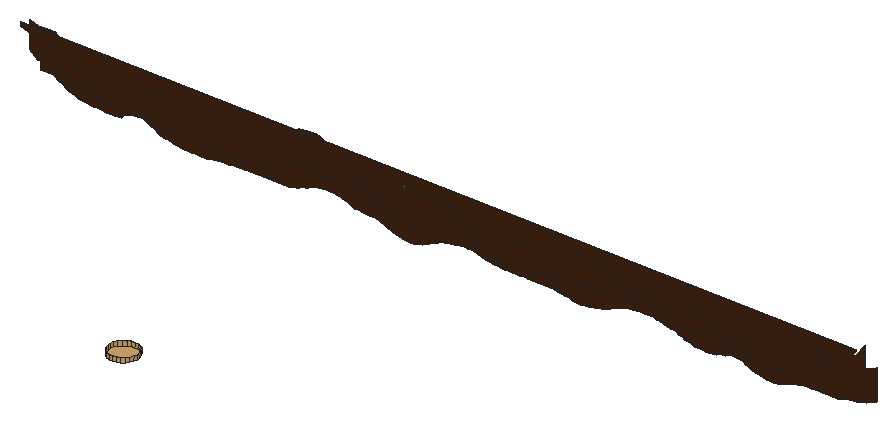
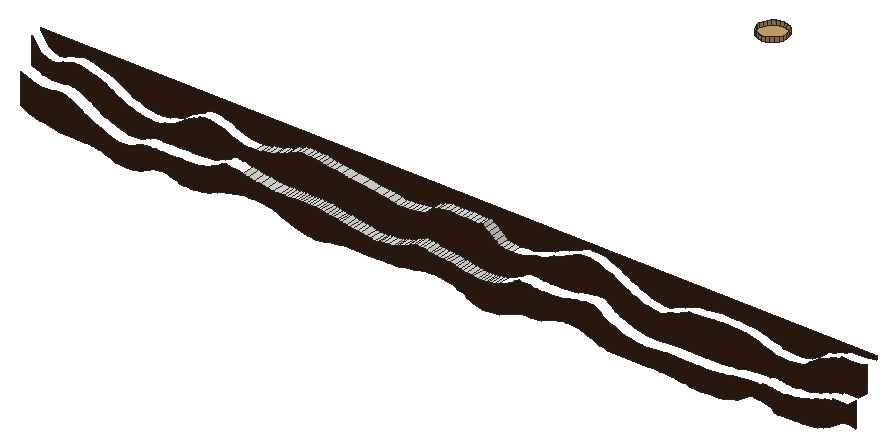
# SketchUp Ruby script. Lengths in inches.
U = 1.inch
M = Sketchup.active_model
def pt(a) = Geom::Point3d.new(a.map { |v| v * U })
def face(e, loops, mat)
  f = e.add_face(loops[0].map { |a| pt(a) })
  loops[1..].each { |l| e.add_face(l.map { |a| pt(a) }).erase! }
  f.material = f.back_material = mat if mat
  f
end
# faces: each face lists its corners as indices into pts; further lists are holes
def faces(e, pts, list, mat = nil) = list.each { |f| face(e, (f[0].is_a?(Array) ? f : [f]).map { |l| l.map { |i| pts[i] } }, mat) }
# xy, xz, yz: faces in a plane at the given z, y or x. An outline is a flat list of corners, or four numbers for a rectangle; further outlines are holes
def ring(l) = l.size == 4 ? [[l[0], l[1]], [l[2], l[1]], [l[2], l[3]], [l[0], l[3]]] : l.each_slice(2).to_a
def flat(e, list, mat, &to3) = list.each { |f| face(e, (f[0].is_a?(Array) ? f : [f]).map { |l| ring(l).map { |u, v| to3.(u, v) } }, mat) }
def xy(e, z, list, mat = nil) = flat(e, list, mat) { |x, y| [x, y, z] }
def xz(e, y, list, mat = nil) = flat(e, list, mat) { |x, z| [x, y, z] }
def yz(e, x, list, mat = nil) = flat(e, list, mat) { |y, z| [x, y, z] }
def lines(e, pts, list) = list.each { |a, b| e.add_line(pt(pts[a]), pt(pts[b])) }
# prism: a flat outline (further loops are holes) pulled along v
def prism(e, loops, v, mat = nil)
  f = face(e, loops, mat); d = Geom::Vector3d.new(v.map { |x| x * U })
  f.pushpull(f.normal.samedirection?(d) ? d.length : -d.length)
end
def box(e, o, s, mat = nil) = prism(e, [[o, [o[0] + s[0], o[1], o[2]], [o[0] + s[0], o[1] + s[1], o[2]], [o[0], o[1] + s[1], o[2]]]], [0, 0, s[2]], mat)
def at(x, y, z, deg = 0) = Geom::Transformation.translation(pt([x, y, z])) * Geom::Transformation.rotation(ORIGIN, Z_AXIS, deg.degrees)
def axes(o, x, y, z) = Geom::Transformation.new([*x, 0, *y, 0, *z, 0, *pt(o).to_a, 1])
def part(name) = M.definitions.add(name)
# library, detail: a bought-in or finely detailed component or shape, given as its bounding box
def library(name, o, s) = part(name).tap { |d| box(d.entities, o, s) }
def detail(e, o, s) = box(e.add_group.entities, o, s)
def put(e, d, t, mat = nil) = e.add_instance(d, t).tap { |i| i.material = mat if mat }
def group(e, t, mat = nil) = e.add_group.tap { |g| g.transformation = t; g.material = mat if mat }.entities
root = M.entities
M.materials.add("[Field Square Tile]").color = [211, 167, 108]
M.materials.add("[Wood Veneer 01]").color = [66, 38, 20]
xy(root,243.05,[[1237.04,2398.8,1237.72,2401.37]])
xy(root,243.07,[[1235.1875,2398.8,1235.77,2401.37]])
xy(root,243.09,[[1231.875,2398.8,1232.4,2401.37],[1232.4,2398.8,1232.92,2401.37],[1232.92,2398.8,1233.58,2401.37],[1233.58,2398.8,1234.03,2401.37]])
xy(root,249.21,[[1204.67,2396.68,1205.56,2398.8]])
xy(root,249.22,[[1206.28,2396.68,1207.1875,2398.8]])
xy(root,249.23,[[1207.83,2396.68,1208.73,2398.8]])
xy(root,250.6875,[[1203.22,2328.39,1202.56,2328.48,1201.94,2328.74,1201.41,2329.14,1201,2329.68,1200.75,2330.29,1200.66,2330.96,1200.75,2331.62,1201,2332.24,1201.41,2332.77,1201.94,2333.18,1202.56,2333.43,1203.22,2333.52,1203.88,2333.43,1204.5,2333.18,1205.03,2332.77,1205.44,2332.24,1205.7,2331.62,1205.78,2330.96,1205.7,2330.29,1205.44,2329.68,1205.03,2329.14,1204.5,2328.74,1203.88,2328.48]],"[Field Square Tile]")
xz(root,2396.68,[[1263.09,244.87,1264,245.01,1264.9375,245.12,1265.7,245.25,1266.46,245.41,1267.09,245.78,1267.89,245.88,1268.6,246.16,1269.2,246.57,1269.99,246.9,1270.59,247.35,1271.26,247.62,1271.85,248.06,1272.61,248.32,1273.72,248.66,1274.5,248.79,1275.36,249.19,1276.03,249.32,1276.96,249.41,1277.81,249.48,1278.56,249.21,1279.2,248.96,1279.9,248.9,1280.7,248.42,1281.41,248.3,1282.12,248.22,1282.9375,248.56,1283.87,249.02,1285.6,251.16,1285.6,251.5,1131.59,251.5,1131.59,250.88,1133.18,250.53,1134.8,250.54,1136.26,250.55,1136.79,250.15,1137.4,249.97,1138.2,249.8,1138.87,249.41,1139.54,249.2,1140.31,249.01,1140.8,248.51,1141.43,248.07,1142.08,247.72,1142.72,247.25,1143.27,246.88,1143.99,246.73,1144.65,246.62,1145.39,246.54,1146.17,246.51,1146.95,246.58,1147.75,246.59,1148.55,246.69,1149.26,247.03,1149.95,247.2,1150.92,247.39,1151.55,247.78,1152.33,247.89,1153.33,248.18,1153.97,248.29,1154.86,248.35,1155.59,248.4,1156.58,248.4375,1157.24,248.46,1158.13,248.47,1158.87,248.48,1159.76,248.49,1160.49,248.39,1161.89,248.28,1162.92,248.15,1163.74,248.11,1164.54,248.08,1165.38,247.66,1166.01,247.46,1166.69,247.08,1167.375,246.94,1168.23,246.66,1168.84,246.35,1169.61,246.05,1170.51,246.13,1171.22,246.29,1172.02,246.41,1172.93,246.55,1173.66,246.92,1174.27,247.12,1174.95,247.31,1175.52,247.71,1176.45,248.03,1177.16,248.46,1177.94,248.82,1178.66,249.37,1179.45,249.5625,1180.35,249.9,1181.27,250.35,1181.93,250.49,1182.74,250.6,1183.76,250.58,1184.4,250.61,1185.02,250.32,1185.71,250.0625,1186.37,249.68,1187.13,249.46,1188.02,248.95,1189.24,248.69,1190.15,248.26,1190.75,247.9,1191.88,247.66,1192.46,247.53,1193.14,247.25,1193.95,246.95,1194.64,246.75,1195.43,246.66,1196.14,246.59,1197.03,246.55,1197.96,246.63,1198.7,246.74,1199.43,246.87,1200.04,247.42,1200.71,247.96,1201.28,248.44,1202.02,248.85,1202.49,249.34,1203.22,249.125,1203.99,249.17,1204.67,249.21,1205.56,249.21,1206.28,249.22,1207.1875,249.22,1207.83,249.23,1208.73,249.23,1209.47,249.24,1210.27,249.14,1210.9,248.82,1211.69,248.54,1212.39,248.04,1213.08,247.48,1213.97,247.29,1214.79,247.15,1215.52,247.05,1216.24,247,1217.15,246.96,1217.875,246.94,1218.79,247.04,1219.85,247.36,1221.03,247.43,1222.68,247.6,1224.66,247.98,1226.86,248.1875,1228.47,248.49,1229.72,248.62,1230.66,248.69,1231.34,248.75,1232,249.09,1232.7,249.18,1233.48,249.13,1234.18,249.17,1234.88,249.18,1235.78,249.29,1236.51,249.21,1237.12,248.8,1237.8125,248.73,1238.59,248.26,1239.29,248.02,1240.09,247.8125,1240.8,247.4,1241.71,247.27,1242.45,247.18,1243.375,246.91,1244.24,246.84,1245.19,246.79,1245.97,246.75,1246.72,246.83,1247.76,247.25,1248.63,247.55,1249.3,247.66,1249.93,248.16,1250.72,248.41,1251.42,248.52,1252.12,248.72,1252.82,248.8,1253.71,248.85,1254.54,248.6875,1255.08,248.26,1255.77,248.06,1256.66,247.55,1257.37,247.19,1258.18,246.63,1258.8125,246.13,1259.4,245.83,1260.08,245.67,1260.95,245.46,1261.66,245.0625,1262.375,244.95]],"[Wood Veneer 01]")
xz(root,2398.8,[[1267.09,241.09,1267.66,241.14,1268.3,241.35,1268.89,241.46,1269.83,241.85,1270.83,242.23,1271.39,242.42,1272.11,242.61,1272.625,242.91,1273,243.14,1273.54,243.52,1274.02,243.71,1274.35,244.02,1274.79,244.21,1275.38,244.57,1275.85,244.76,1276.47,245.125,1276.97,245.32,1277.45,245.41,1278,245.48,1278.49,245.59,1279.02,245.55,1279.63,245.35,1280.12,245.31,1280.67,245.27,1281.23,245.24,1281.79,245.22,1282.35,245.34,1282.98,245.42,1283.5625,245.52,1283.94,245.76,1284.41,245.9,1285.6,246.43,1285.6,251.16,1283.87,249.02,1282.9375,248.56,1282.12,248.22,1281.41,248.3,1280.7,248.42,1279.9,248.9,1279.2,248.96,1278.56,249.21,1277.81,249.48,1276.96,249.41,1276.03,249.32,1275.36,249.19,1274.5,248.79,1273.72,248.66,1272.61,248.32,1271.85,248.06,1271.26,247.62,1270.59,247.35,1269.99,246.9,1269.2,246.57,1268.6,246.16,1267.89,245.88,1267.09,245.78,1266.46,245.41,1265.7,245.25,1264.9375,245.12,1264,245.01,1263.09,244.87,1262.375,244.95,1261.66,245.0625,1260.95,245.46,1260.08,245.67,1259.4,245.83,1258.8125,246.13,1258.18,246.63,1257.37,247.19,1256.66,247.55,1255.77,248.06,1255.08,248.26,1254.54,248.6875,1253.71,248.85,1252.82,248.8,1252.12,248.72,1251.42,248.52,1250.72,248.41,1249.93,248.16,1249.3,247.66,1248.63,247.55,1247.76,247.25,1246.72,246.83,1245.97,246.75,1245.19,246.79,1244.24,246.84,1243.375,246.91,1242.45,247.18,1241.71,247.27,1240.8,247.4,1240.09,247.8125,1239.29,248.02,1238.59,248.26,1237.8125,248.73,1237.12,248.8,1236.51,249.21,1235.78,249.29,1234.88,249.18,1234.18,249.17,1233.48,249.13,1232.7,249.18,1232,249.09,1231.34,248.75,1230.66,248.69,1229.72,248.62,1228.47,248.49,1226.86,248.1875,1224.66,247.98,1222.68,247.6,1221.03,247.43,1219.85,247.36,1218.79,247.04,1217.875,246.94,1217.15,246.96,1216.24,247,1215.52,247.05,1214.79,247.15,1213.97,247.29,1213.08,247.48,1212.39,248.04,1211.69,248.54,1210.9,248.82,1210.27,249.14,1209.47,249.24,1208.73,249.23,1207.83,249.23,1207.1875,249.22,1206.28,249.22,1205.56,249.21,1204.67,249.21,1203.99,249.17,1203.22,249.125,1202.49,249.34,1202.02,248.85,1201.28,248.44,1200.71,247.96,1200.04,247.42,1199.43,246.87,1198.7,246.74,1197.96,246.63,1197.03,246.55,1196.14,246.59,1195.43,246.66,1194.64,246.75,1193.95,246.95,1193.14,247.25,1192.46,247.53,1191.88,247.66,1190.75,247.9,1190.15,248.26,1189.24,248.69,1188.02,248.95,1187.13,249.46,1186.37,249.68,1185.71,250.0625,1185.02,250.32,1184.4,250.61,1183.76,250.58,1182.74,250.6,1181.93,250.49,1181.27,250.35,1180.35,249.9,1179.45,249.5625,1178.66,249.37,1177.94,248.82,1177.16,248.46,1176.45,248.03,1175.52,247.71,1174.95,247.31,1174.27,247.12,1173.66,246.92,1172.93,246.55,1172.02,246.41,1171.22,246.29,1170.51,246.13,1169.61,246.05,1168.84,246.35,1168.23,246.66,1167.375,246.94,1166.69,247.08,1166.01,247.46,1165.38,247.66,1164.54,248.08,1163.74,248.11,1162.92,248.15,1161.89,248.28,1160.49,248.39,1159.76,248.49,1158.87,248.48,1158.13,248.47,1157.24,248.46,1156.58,248.4375,1155.59,248.4,1154.86,248.35,1153.97,248.29,1153.33,248.18,1152.33,247.89,1151.55,247.78,1150.92,247.39,1149.95,247.2,1149.26,247.03,1148.55,246.69,1147.75,246.59,1146.95,246.58,1146.17,246.51,1145.39,246.54,1144.65,246.62,1143.99,246.73,1143.27,246.88,1142.72,247.25,1142.08,247.72,1141.43,248.07,1140.8,248.51,1140.31,249.01,1139.54,249.2,1138.87,249.41,1138.2,249.8,1137.4,249.97,1136.79,250.15,1136.26,250.55,1134.8,250.54,1133.18,250.53,1131.59,250.88,1131.59,246.2,1133.16,244.96,1134.55,244.9375,1135.8,244.92,1136.02,244.61,1136.58,244.54,1137.34,244.41,1138.01,244.11,1138.53,243.95,1139.19,243.79,1139.71,243.48,1140.35,243.3,1140.9375,243.14,1141.42,243.06,1142.14,242.85,1142.72,242.78,1143.53,242.73,1144.07,242.68,1144.74,242.51,1145.26,242.46,1145.8,242.58,1146.43,242.57,1147.06,242.81,1147.63,242.86,1148.19,242.89,1148.83,242.92,1149.26,242.625,1149.87,242.65,1150.42,242.62,1151.05,242.58,1151.61,242.57,1152.25,242.48,1152.91,242.38,1153.57,242.34,1154.24,242.24,1155.41,241.96,1156.18,241.89,1157,241.83,1157.6,241.78,1158.37,241.75,1158.82,241.74,1159.37,241.72,1160.63,241.7,1161.36,241.69,1162.03,241.68,1162.62,241.68,1163.11,241.67,1163.8125,241.74,1164.38,241.75,1166.38,241.75,1166.87,241.67,1167.4,241.66,1168.01,241.57,1168.55,241.53,1169.17,241.51,1169.72,241.49,1170.42,241.48,1171.08,241.47,1171.65,241.46,1172.36,241.6,1173.09,241.85,1173.76,241.91,1174.66,242.1,1175.43,242.46,1176.13,242.78,1176.9,242.97,1177.43,243.23,1177.83,243.48,1178.35,243.72,1178.6875,244.12,1179.16,244.39,1179.64,244.73,1180.125,244.87,1180.71,244.95,1181.39,245.01,1182.04,244.81,1182.61,244.7,1183.09,244.67,1183.7,244.55,1184.24,244.51,1184.7,244.25,1185.45,244.11,1186.01,244.04,1186.63,243.99,1187.35,243.95,1187.85,243.93,1188.54,243.91,1189.11,243.89,1189.81,243.88,1190.46,243.94,1191.1,243.95,1191.66,244.1,1192.29,244.13,1192.77,244.15,1193.29,244.17,1193.81,244.18,1194.41,243.8,1194.95,243.43,1195.56,243.09,1195.95,242.875,1196.45,242.68,1197.04,242.51,1197.55,242.21,1198.15,242.11,1198.83,241.96,1199.39,241.89,1199.85,241.85,1200.37,241.8125,1200.88,241.79,1201.46,241.78,1202.13,241.91,1202.6,241.93,1203.27,242.09,1204.04,242.2,1204.54,242.24,1205.15,242.42,1205.7,242.47,1206.45,242.71,1207.09,242.78,1207.57,242.82,1208.26,242.85,1208.96,242.87,1209.51,243.02,1210.13,243.05,1210.68,243.29,1211.36,243.35,1211.91,243.39,1212.51,243.42,1213.28,243.14,1213.85,242.9375,1214.4,242.65,1215.02,242.39,1215.78,242.14,1216.42,241.89,1216.91,241.78,1217.96,241.63,1218.73,241.56,1219.33,241.51,1219.78,241.48,1220.3,241.46,1221.17,241.51,1221.89,241.59,1222.83,241.82,1223.61,241.87,1224.375,241.98,1224.99,242.02,1225.64,242.19,1226.34,242.38,1226.83,242.4375,1227.35,242.48,1228.01,242.58,1228.54,242.61,1229.125,242.77,1229.58,242.95,1230.14,243.01,1230.65,243.05,1231.22,243.08,1231.875,243.09,1234.03,243.09,1234.6,243.08,1235.1875,243.07,1235.77,243.07,1236.43,243.0625,1237.04,243.05,1237.72,243.05,1238.99,243.1,1240.16,243.17,1241.3,243.4,1242.5625,243.52,1243.69,243.71,1244.59,243.99,1245.29,244.08,1245.99,244.21,1246.57,244.27,1247.11,244.3,1247.78,244.39,1248.375,244.19,1248.75,243.88,1249.23,243.59,1249.78,243.33,1250.33,243.22,1250.82,242.92,1251.3,242.75,1251.86,242.6,1252.42,242.52,1252.98,242.47,1253.5625,242.43,1254.14,242.4,1254.72,242.39,1255.3,242.37,1255.88,242.36,1256.47,242.35,1257.63,242.33,1258.21,242.33,1258.93,242.32,1259.4,242.3125,1260.04,242.3,1260.71,242.3,1261.16,242.29,1261.8,242.28,1262.3125,242.28,1262.94,242.2,1263.52,241.97,1264.09,241.84,1264.6,241.57,1265.02,241.33,1265.49,241.24,1266.02,241.17,1266.49,241.12]],"[Wood Veneer 01]")
xz(root,2401.37,[[1200.45,236.98,1201.13,237.22,1201.98,237.43,1202.6,237.74,1203.3,238.02,1203.74,238.375,1204.3,238.51,1204.9375,238.76,1205.58,239.12,1206.16,239.22,1207.16,239.31,1207.97,239.54,1208.46,239.6,1209.08,239.65,1209.67,239.69,1210.23,239.7,1210.96,239.72,1211.57,239.56,1212.24,239.44,1213.09,239.16,1213.64,239.07,1214.41,238.93,1215.29,238.78,1215.77,238.73,1216.44,238.6875,1217.13,238.66,1217.8,238.65,1218.58,238.64,1219.2,238.63,1219.89,238.625,1220.75,238.625,1221.31,238.62,1226.2,238.62,1226.89,238.45,1227.65,238.25,1228.27,238.19,1229.04,238.15,1229.67,237.86,1230.44,237.79,1231.15,237.74,1232.02,237.87,1232.67,237.88,1233.79,238.14,1235.01,238.46,1235.76,238.72,1236.64,239.08,1237.43,239.375,1238.17,239.75,1238.82,239.97,1239.44,240.17,1240.12,240.27,1240.8,240.33,1241.49,240.37,1242.18,240.4,1242.875,240.41,1243.4,240.42,1243.98,240.43,1244.55,240.43,1245.2,240.27,1245.78,240.23,1246.43,239.96,1247.1875,239.8,1247.8,239.65,1248.5625,239.5,1249.1875,239.18,1249.87,239.01,1250.39,238.67,1250.96,238.56,1251.62,238.48,1252.1875,238.26,1252.76,238.19,1253.58,238.15,1254.11,238.11,1254.78,238.18,1255.46,238.18,1256.14,238.27,1256.66,238.55,1257.32,238.61,1257.91,238.66,1258.48,239.04,1259.22,239.125,1259.9,239.02,1260.59,238.96,1261.11,238.86,1261.61,238.57,1262.16,238.33,1262.87,238,1263.7,237.71,1264.24,237.59,1264.84,237.51,1265.43,237.45,1266,237.42,1266.73,237.4,1267.41,237.47,1268.01,237.5625,1268.7,237.84,1269.38,238.08,1270.07,238.33,1270.6,238.51,1271.17,238.6,1271.83,238.74,1272.41,238.8,1272.98,238.83,1273.72,238.86,1274.48,238.875,1275.02,238.88,1275.7,238.89,1276.38,238.89,1277.14,238.9,1278.53,238.9,1279.16,239.15,1279.93,239.28,1280.73,239.42,1281.45,239.49,1282,239.53,1282.6875,239.81,1283.21,239.96,1283.77,240.1,1285.6,240.89,1285.6,246.43,1284.41,245.9,1283.94,245.76,1283.5625,245.52,1282.98,245.42,1282.35,245.34,1281.79,245.22,1281.23,245.24,1280.67,245.27,1280.12,245.31,1279.63,245.35,1279.02,245.55,1278.49,245.59,1278,245.48,1277.45,245.41,1276.97,245.32,1276.47,245.125,1275.85,244.76,1275.38,244.57,1274.79,244.21,1274.35,244.02,1274.02,243.71,1273.54,243.52,1273,243.14,1272.625,242.91,1272.11,242.61,1271.39,242.42,1270.83,242.23,1269.83,241.85,1268.89,241.46,1268.3,241.35,1267.66,241.14,1267.09,241.09,1266.49,241.12,1266.02,241.17,1265.49,241.24,1265.02,241.33,1264.6,241.57,1264.09,241.84,1263.52,241.97,1262.94,242.2,1262.3125,242.28,1261.8,242.28,1261.16,242.29,1260.71,242.3,1260.04,242.3,1259.4,242.3125,1258.93,242.32,1258.21,242.33,1257.63,242.33,1256.47,242.35,1255.88,242.36,1255.3,242.37,1254.72,242.39,1254.14,242.4,1253.5625,242.43,1252.98,242.47,1252.42,242.52,1251.86,242.6,1251.3,242.75,1250.82,242.92,1250.33,243.22,1249.78,243.33,1249.23,243.59,1248.75,243.88,1248.375,244.19,1247.78,244.39,1247.11,244.3,1246.57,244.27,1245.99,244.21,1245.29,244.08,1244.59,243.99,1243.69,243.71,1242.5625,243.52,1241.3,243.4,1240.16,243.17,1238.99,243.1,1237.72,243.05,1237.04,243.05,1236.43,243.0625,1235.77,243.07,1235.1875,243.07,1234.6,243.08,1234.03,243.09,1231.875,243.09,1231.22,243.08,1230.65,243.05,1230.14,243.01,1229.58,242.95,1229.125,242.77,1228.54,242.61,1228.01,242.58,1227.35,242.48,1226.83,242.4375,1226.34,242.38,1225.64,242.19,1224.99,242.02,1224.375,241.98,1223.61,241.87,1222.83,241.82,1221.89,241.59,1221.17,241.51,1220.3,241.46,1219.78,241.48,1219.33,241.51,1218.73,241.56,1217.96,241.63,1216.91,241.78,1216.42,241.89,1215.78,242.14,1215.02,242.39,1214.4,242.65,1213.85,242.9375,1213.28,243.14,1212.51,243.42,1211.91,243.39,1211.36,243.35,1210.68,243.29,1210.13,243.05,1209.51,243.02,1208.96,242.87,1208.26,242.85,1207.57,242.82,1207.09,242.78,1206.45,242.71,1205.7,242.47,1205.15,242.42,1204.54,242.24,1204.04,242.2,1203.27,242.09,1202.6,241.93,1202.13,241.91,1201.46,241.78,1200.88,241.79,1200.37,241.8125,1199.85,241.85,1199.39,241.89,1198.83,241.96,1198.15,242.11,1197.55,242.21,1197.04,242.51,1196.45,242.68,1195.95,242.875,1195.56,243.09,1194.95,243.43,1194.41,243.8,1193.81,244.18,1193.29,244.17,1192.77,244.15,1192.29,244.13,1191.66,244.1,1191.1,243.95,1190.46,243.94,1189.81,243.88,1189.11,243.89,1188.54,243.91,1187.85,243.93,1187.35,243.95,1186.63,243.99,1186.01,244.04,1185.45,244.11,1184.7,244.25,1184.24,244.51,1183.7,244.55,1183.09,244.67,1182.61,244.7,1182.04,244.81,1181.39,245.01,1180.71,244.95,1180.125,244.87,1179.64,244.73,1179.16,244.39,1178.6875,244.12,1178.35,243.72,1177.83,243.48,1177.43,243.23,1176.9,242.97,1176.13,242.78,1175.43,242.46,1174.66,242.1,1173.76,241.91,1173.09,241.85,1172.36,241.6,1171.65,241.46,1171.08,241.47,1170.42,241.48,1169.72,241.49,1169.17,241.51,1168.55,241.53,1168.01,241.57,1167.4,241.66,1166.87,241.67,1166.38,241.75,1164.38,241.75,1163.8125,241.74,1163.11,241.67,1162.62,241.68,1162.03,241.68,1161.36,241.69,1160.63,241.7,1159.37,241.72,1158.82,241.74,1158.37,241.75,1157.6,241.78,1157,241.83,1156.18,241.89,1155.41,241.96,1154.24,242.24,1153.57,242.34,1152.91,242.38,1152.25,242.48,1151.61,242.57,1151.05,242.58,1150.42,242.62,1149.87,242.65,1149.26,242.625,1148.83,242.92,1148.19,242.89,1147.63,242.86,1147.06,242.81,1146.43,242.57,1145.8,242.58,1145.26,242.46,1144.74,242.51,1144.07,242.68,1143.53,242.73,1142.72,242.78,1142.14,242.85,1141.42,243.06,1140.9375,243.14,1140.35,243.3,1139.71,243.48,1139.19,243.79,1138.53,243.95,1138.01,244.11,1137.34,244.41,1136.58,244.54,1136.02,244.61,1135.8,244.92,1134.55,244.9375,1133.16,244.96,1131.59,246.2,1131.59,241.52,1132.8,241.69,1134.07,241.55,1135.09,240.85,1135.63,240.59,1136.23,240.2,1137.02,239.86,1137.47,239.64,1138.03,239.52,1138.54,239.19,1139.32,239.09,1140.01,239.03,1140.69,238.97,1141.39,238.94,1142.09,238.93,1142.78,238.92,1143.82,238.82,1144.33,238.8,1145.2,238.79,1145.94,238.77,1146.47,238.9375,1147.03,239.55,1147.61,239.69,1148.16,239.88,1148.89,239.99,1149.48,240.05,1150.14,240.09,1150.83,240.11,1151.53,239.71,1151.99,239.38,1152.57,239.11,1153.15,238.74,1153.8,238.43,1154.71,238.31,1155.18,238.21,1156.12,237.9,1156.78,237.82,1157.47,237.76,1158.18,237.71,1158.79,237.68,1159.39,237.67,1160.14,237.66,1160.83,237.65,1162.14,237.65,1162.81,237.89,1163.57,237.94,1164.1875,237.98,1165.04,238.1,1165.59,238.13,1166.35,238.15,1166.98,238.26,1167.73,238.28,1168.36,238.3,1169.21,238.32,1169.93,238.33,1171.16,238.33,1171.84,238.34,1177.41,238.34,1177.92,238.59,1178.74,238.72,1179.43,238.86,1179.94,239.18,1180.53,239.35,1181.09,239.52,1181.64,239.85,1182.28,240.03,1182.9375,240.12,1183.61,240.19,1184.375,240.23,1185.08,240.25,1185.7,240.27,1186.48,240.11,1187.11,239.92,1187.8,239.7,1188.33,239.53,1188.91,239.29,1189.57,239.04,1190.15,238.94,1190.72,238.875,1191.47,238.83,1192.23,238.8,1192.77,238.79,1193.44,238.78,1194.22,238.43,1195,238.28,1195.5625,237.96,1196.5,237.68,1197.17,237.33,1197.7,237.2,1198.39,237.11,1199.15,237.04,1199.84,237.01]],"[Wood Veneer 01]")
p = [[1218.73,2398.8,241.56],[1218.73,2401.37,241.56],[1219.33,2401.37,241.51],[1219.33,2398.8,241.51],[1219.78,2401.37,241.48],[1219.78,2398.8,241.48],
  [1220.3,2401.37,241.46],[1220.3,2398.8,241.46],[1221.17,2401.37,241.51],[1221.17,2398.8,241.51],[1221.89,2401.37,241.59],[1221.89,2398.8,241.59],
  [1216.91,2398.8,241.78],[1216.91,2401.37,241.78],[1217.96,2401.37,241.63],[1217.96,2398.8,241.63],[1222.83,2401.37,241.82],[1222.83,2398.8,241.82],
  [1199.39,2398.8,241.89],[1199.39,2401.37,241.89],[1199.85,2401.37,241.85],[1199.85,2398.8,241.85],[1200.37,2401.37,241.8125],[1200.37,2398.8,241.8125],
  [1200.88,2401.37,241.79],[1200.88,2398.8,241.79],[1201.46,2401.37,241.78],[1201.46,2398.8,241.78],[1202.13,2401.37,241.91],[1202.13,2398.8,241.91],
  [1216.42,2398.8,241.89],[1216.42,2401.37,241.89],[1223.61,2401.37,241.87],[1223.61,2398.8,241.87],[1198.83,2398.8,241.96],[1198.83,2401.37,241.96],
  [1202.6,2401.37,241.93],[1202.6,2398.8,241.93],[1203.27,2401.37,242.09],[1203.27,2398.8,242.09],[1215.78,2398.8,242.14],[1215.78,2401.37,242.14],
  [1224.375,2401.37,241.98],[1224.375,2398.8,241.98],[1198.15,2398.8,242.11],[1198.15,2401.37,242.11],[1224.99,2401.37,242.02],[1224.99,2398.8,242.02],
  [1225.64,2401.37,242.19],[1225.64,2398.8,242.19],[1197.55,2398.8,242.21],[1197.55,2401.37,242.21],[1204.04,2401.37,242.2],[1204.04,2398.8,242.2],
  [1215.02,2398.8,242.39],[1215.02,2401.37,242.39],[1204.54,2401.37,242.24],[1204.54,2398.8,242.24],[1205.15,2401.37,242.42],[1205.15,2398.8,242.42],
  [1226.34,2401.37,242.38],[1226.34,2398.8,242.38],[1205.7,2401.37,242.47],[1205.7,2398.8,242.47],[1214.4,2398.8,242.65],[1214.4,2401.37,242.65],
  [1226.83,2401.37,242.4375],[1226.83,2398.8,242.4375],[1227.35,2401.37,242.48],[1227.35,2398.8,242.48],[1206.45,2401.37,242.71],[1206.45,2398.8,242.71],
  [1228.01,2401.37,242.58],[1228.01,2398.8,242.58],[1213.85,2398.8,242.9375],[1213.85,2401.37,242.9375],[1228.54,2401.37,242.61],[1228.54,2398.8,242.61],
  [1229.125,2401.37,242.77],[1229.125,2398.8,242.77],[1207.09,2401.37,242.78],[1207.09,2398.8,242.78],[1207.57,2401.37,242.82],[1207.57,2398.8,242.82],
  [1208.26,2401.37,242.85],[1208.26,2398.8,242.85],[1229.58,2401.37,242.95],[1229.58,2398.8,242.95],[1208.96,2401.37,242.87],[1208.96,2398.8,242.87],
  [1209.51,2401.37,243.02],[1209.51,2398.8,243.02],[1213.28,2398.8,243.14],[1213.28,2401.37,243.14],[1210.13,2401.37,243.05],[1210.13,2398.8,243.05],
  [1230.14,2401.37,243.01],[1230.14,2398.8,243.01],[1230.65,2401.37,243.05],[1230.65,2398.8,243.05],[1231.22,2401.37,243.08],[1231.22,2398.8,243.08],
  [1237.72,2398.8,243.05],[1237.72,2401.37,243.05],[1238.99,2401.37,243.1],[1238.99,2398.8,243.1],[1210.68,2401.37,243.29],[1210.68,2398.8,243.29],
  [1212.51,2398.8,243.42],[1212.51,2401.37,243.42],[1231.875,2401.37,243.09],[1231.875,2398.8,243.09],[1234.03,2398.8,243.09],[1234.03,2401.37,243.09],
  [1234.6,2401.37,243.08],[1234.6,2398.8,243.08],[1235.1875,2401.37,243.07],[1235.1875,2398.8,243.07],[1235.77,2398.8,243.07],[1235.77,2401.37,243.07],
  [1236.43,2401.37,243.0625],[1236.43,2398.8,243.0625],[1237.04,2401.37,243.05],[1237.04,2398.8,243.05],[1240.16,2401.37,243.17],[1240.16,2398.8,243.17],
  [1241.3,2401.37,243.4],[1241.3,2398.8,243.4],[1211.36,2401.37,243.35],[1211.36,2398.8,243.35],[1211.91,2401.37,243.39],[1211.91,2398.8,243.39],
  [1242.5625,2401.37,243.52],[1242.5625,2398.8,243.52],[1243.69,2401.37,243.71],[1243.69,2398.8,243.71],[1244.59,2401.37,243.99],[1244.59,2398.8,243.99],
  [1197.03,2396.68,246.55],[1197.03,2398.8,246.55],[1197.96,2398.8,246.63],[1197.96,2396.68,246.63],[1198.7,2398.8,246.74],[1198.7,2396.68,246.74],
  [1199.43,2398.8,246.87],[1199.43,2396.68,246.87],[1243.375,2396.68,246.91],[1243.375,2398.8,246.91],[1244.24,2398.8,246.84],[1244.24,2396.68,246.84],
  [1200.04,2398.8,247.42],[1200.04,2396.68,247.42],[1217.15,2396.68,246.96],[1217.15,2398.8,246.96],[1217.875,2398.8,246.94],[1217.875,2396.68,246.94],
  [1218.79,2398.8,247.04],[1218.79,2396.68,247.04],[1242.45,2396.68,247.18],[1242.45,2398.8,247.18],[1214.79,2396.68,247.15],[1214.79,2398.8,247.15],
  [1215.52,2398.8,247.05],[1215.52,2396.68,247.05],[1216.24,2398.8,247],[1216.24,2396.68,247],[1219.85,2398.8,247.36],[1219.85,2396.68,247.36],
  [1213.97,2396.68,247.29],[1213.97,2398.8,247.29],[1241.71,2396.68,247.27],[1241.71,2398.8,247.27],[1213.08,2396.68,247.48],[1213.08,2398.8,247.48],
  [1240.8,2396.68,247.4],[1240.8,2398.8,247.4],[1200.71,2398.8,247.96],[1200.71,2396.68,247.96],[1221.03,2398.8,247.43],[1221.03,2396.68,247.43],
  [1222.68,2398.8,247.6],[1222.68,2396.68,247.6],[1240.09,2396.68,247.8125],[1240.09,2398.8,247.8125],[1212.39,2396.68,248.04],[1212.39,2398.8,248.04],
  [1224.66,2398.8,247.98],[1224.66,2396.68,247.98],[1239.29,2396.68,248.02],[1239.29,2398.8,248.02],[1201.28,2398.8,248.44],[1201.28,2396.68,248.44],
  [1211.69,2396.68,248.54],[1211.69,2398.8,248.54],[1226.86,2398.8,248.1875],[1226.86,2396.68,248.1875],[1238.59,2396.68,248.26],[1238.59,2398.8,248.26],
  [1228.47,2398.8,248.49],[1228.47,2396.68,248.49],[1237.8125,2396.68,248.73],[1237.8125,2398.8,248.73],[1202.02,2398.8,248.85],[1202.02,2396.68,248.85],
  [1210.9,2396.68,248.82],[1210.9,2398.8,248.82],[1229.72,2398.8,248.62],[1229.72,2396.68,248.62],[1230.66,2398.8,248.69],[1230.66,2396.68,248.69],
  [1231.34,2398.8,248.75],[1231.34,2396.68,248.75],[1237.12,2396.68,248.8],[1237.12,2398.8,248.8],[1210.27,2396.68,249.14],[1210.27,2398.8,249.14],
  [1232,2398.8,249.09],[1232,2396.68,249.09],[1236.51,2396.68,249.21],[1236.51,2398.8,249.21],[1202.49,2398.8,249.34],[1202.49,2396.68,249.34],
  [1203.22,2398.8,249.125],[1203.22,2396.68,249.125],[1203.99,2398.8,249.17],[1203.99,2396.68,249.17],[1209.47,2396.68,249.24],[1209.47,2398.8,249.24],
  [1232.7,2398.8,249.18],[1232.7,2396.68,249.18],[1233.48,2398.8,249.13],[1233.48,2396.68,249.13],[1234.18,2398.8,249.17],[1234.18,2396.68,249.17],
  [1204.67,2398.8,249.21],[1204.67,2396.68,249.21],[1205.56,2396.68,249.21],[1205.56,2398.8,249.21],[1206.28,2398.8,249.22],[1206.28,2396.68,249.22],
  [1207.1875,2396.68,249.22],[1207.1875,2398.8,249.22],[1207.83,2398.8,249.23],[1207.83,2396.68,249.23],[1208.73,2396.68,249.23],[1208.73,2398.8,249.23],
  [1234.88,2398.8,249.18],[1234.88,2396.68,249.18],[1235.78,2398.8,249.29],[1235.78,2396.68,249.29],[1203.22,2328.39,251.5],[1202.56,2328.48,251.5],
  [1202.56,2328.48,250.6875],[1203.22,2328.39,250.6875],[1203.88,2328.48,251.5],[1203.88,2328.48,250.6875],[1201.94,2328.74,251.5],[1201.94,2328.74,250.6875],
  [1204.5,2328.74,251.5],[1204.5,2328.74,250.6875],[1201.41,2329.14,251.5],[1201.41,2329.14,250.6875],[1205.03,2329.14,251.5],[1205.03,2329.14,250.6875],
  [1201,2329.68,251.5],[1201,2329.68,250.6875],[1205.44,2329.68,251.5],[1205.44,2329.68,250.6875],[1200.75,2330.29,251.5],[1200.75,2330.29,250.6875],
  [1205.7,2330.29,251.5],[1205.7,2330.29,250.6875],[1200.66,2330.96,251.5],[1200.66,2330.96,250.6875],[1205.78,2330.96,251.5],[1205.78,2330.96,250.6875],
  [1200.75,2331.62,251.5],[1200.75,2331.62,250.6875],[1205.7,2331.62,251.5],[1205.7,2331.62,250.6875],[1201,2332.24,251.5],[1201,2332.24,250.6875],
  [1205.44,2332.24,251.5],[1205.44,2332.24,250.6875],[1201.41,2332.77,251.5],[1201.41,2332.77,250.6875],[1205.03,2332.77,251.5],[1205.03,2332.77,250.6875],
  [1201.94,2333.18,251.5],[1201.94,2333.18,250.6875],[1204.5,2333.18,251.5],[1204.5,2333.18,250.6875],[1202.56,2333.43,251.5],[1202.56,2333.43,250.6875],
  [1203.88,2333.43,251.5],[1203.88,2333.43,250.6875],[1203.22,2333.52,251.5],[1203.22,2333.52,250.6875]]
faces(root,p,[[0,1,2,3],[3,2,4,5],[5,4,6,7],[7,6,8,9],[9,8,10,11],[12,13,14,15],[15,14,1,0],[11,10,16,17],
  [18,19,20,21],[21,20,22,23],[23,22,24,25],[25,24,26,27],[27,26,28,29],[30,31,13,12],[17,16,32,33],[34,35,19,18],
  [29,28,36,37],[37,36,38,39],[40,41,31,30],[33,32,42,43],[44,45,35,34],[43,42,46,47],[47,46,48,49],[50,51,45,44],
  [39,38,52,53],[54,55,41,40],[53,52,56,57],[57,56,58,59],[49,48,60,61],[59,58,62,63],[64,65,55,54],[61,60,66,67],
  [67,66,68,69],[63,62,70,71],[69,68,72,73],[74,75,65,64],[73,72,76,77],[77,76,78,79],[71,70,80,81],[81,80,82,83],
  [83,82,84,85],[79,78,86,87],[85,84,88,89],[89,88,90,91],[92,93,75,74],[91,90,94,95],[87,86,96,97],[97,96,98,99],
  [99,98,100,101],[102,103,104,105],[95,94,106,107],[108,109,93,92],[101,100,110,111],[112,113,114,115],[115,114,116,117],[118,119,120,121],
  [121,120,122,123],[105,104,124,125],[125,124,126,127],[107,106,128,129],[129,128,130,131],[131,130,109,108],[127,126,132,133],[133,132,134,135],
  [135,134,136,137],[138,139,140,141],[141,140,142,143],[143,142,144,145],[146,147,148,149],[145,144,150,151],[152,153,154,155],[155,154,156,157],
  [158,159,147,146],[160,161,162,163],[163,162,164,165],[165,164,153,152],[157,156,166,167],[168,169,161,160],[170,171,159,158],[172,173,169,168],
  [174,175,171,170],[151,150,176,177],[167,166,178,179],[179,178,180,181],[182,183,175,174],[184,185,173,172],[181,180,186,187],[188,189,183,182],
  [177,176,190,191],[192,193,185,184],[187,186,194,195],[196,197,189,188],[195,194,198,199],[200,201,197,196],[191,190,202,203],[204,205,193,192],
  [199,198,206,207],[207,206,208,209],[209,208,210,211],[212,213,201,200],[214,215,205,204],[211,210,216,217],[218,219,213,212],[203,202,220,221],
  [221,220,222,223],[223,222,224,225],[226,227,215,214],[217,216,228,229],[229,228,230,231],[231,230,232,233],[225,224,234,235],[236,237,238,239],
  [240,241,242,243],[244,245,227,226],[233,232,246,247],[247,246,248,249],[249,248,219,218]])
faces(root,p,[[250,251,252,253],[254,250,253,255],[251,256,257,252],[258,254,255,259],[256,260,261,257],[262,258,259,263],[260,264,265,261],[266,262,263,267],
  [264,268,269,265],[270,266,267,271],[268,272,273,269],[274,270,271,275],[272,276,277,273],[278,274,275,279],[276,280,281,277],[282,278,279,283],
  [280,284,285,281],[286,282,283,287],[284,288,289,285],[290,286,287,291],[288,292,293,289],[294,290,291,295],[292,296,297,293],[296,294,295,297]],"[Field Square Tile]")
